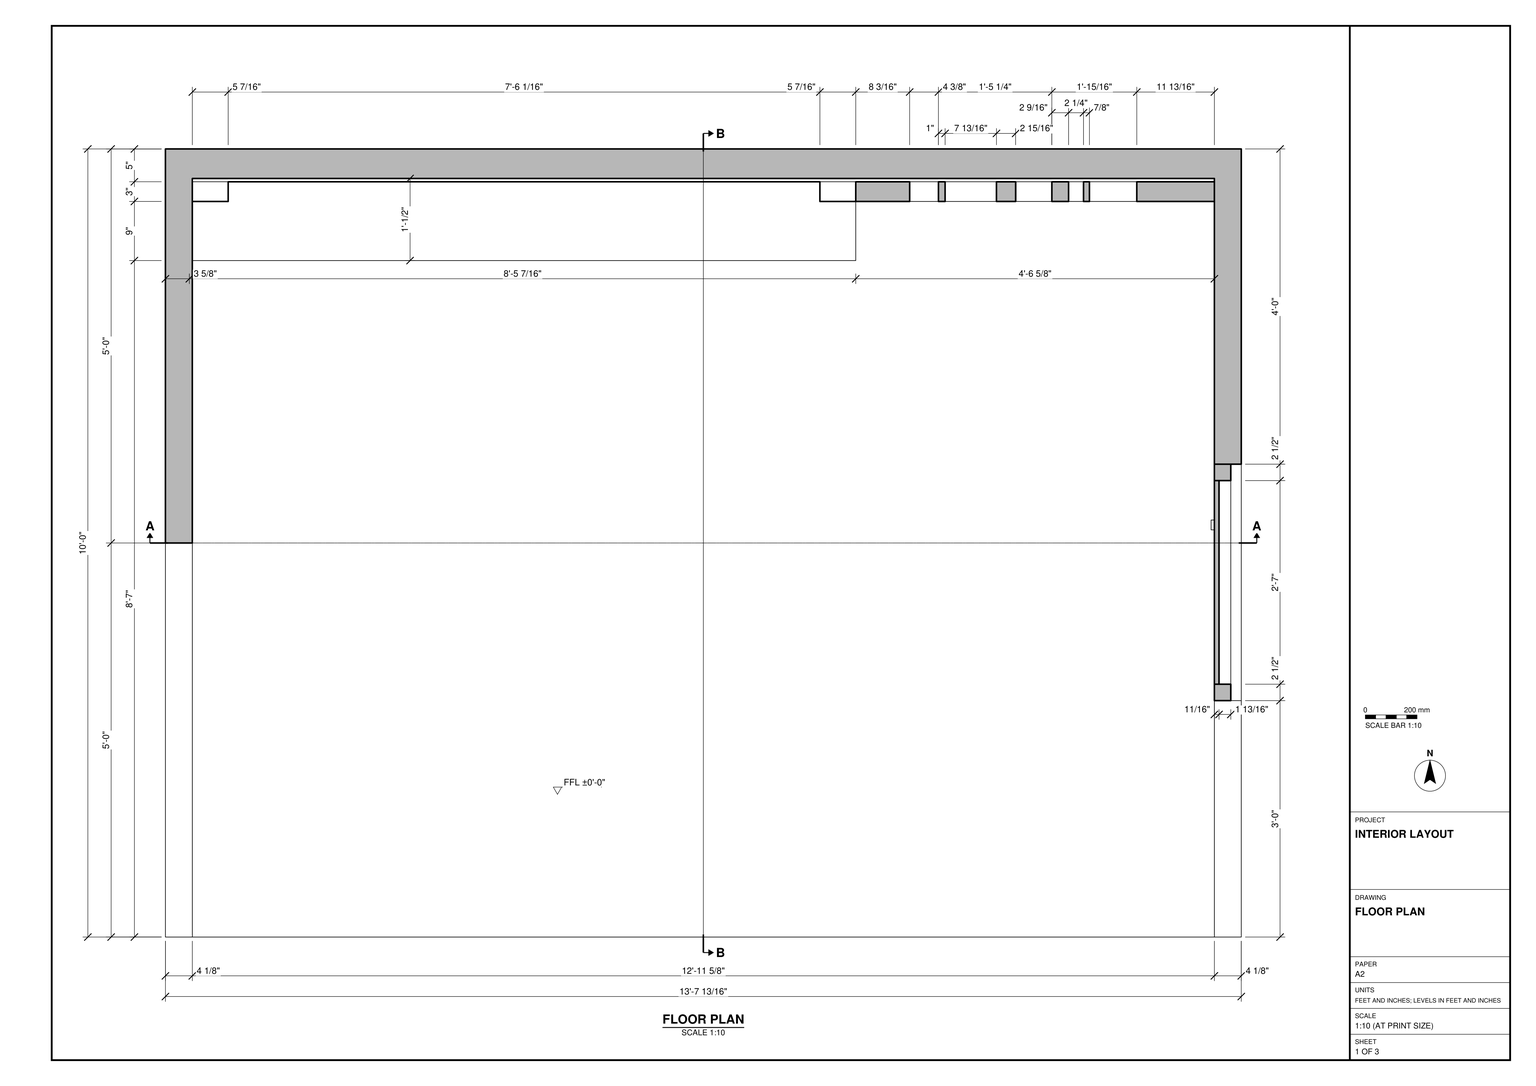
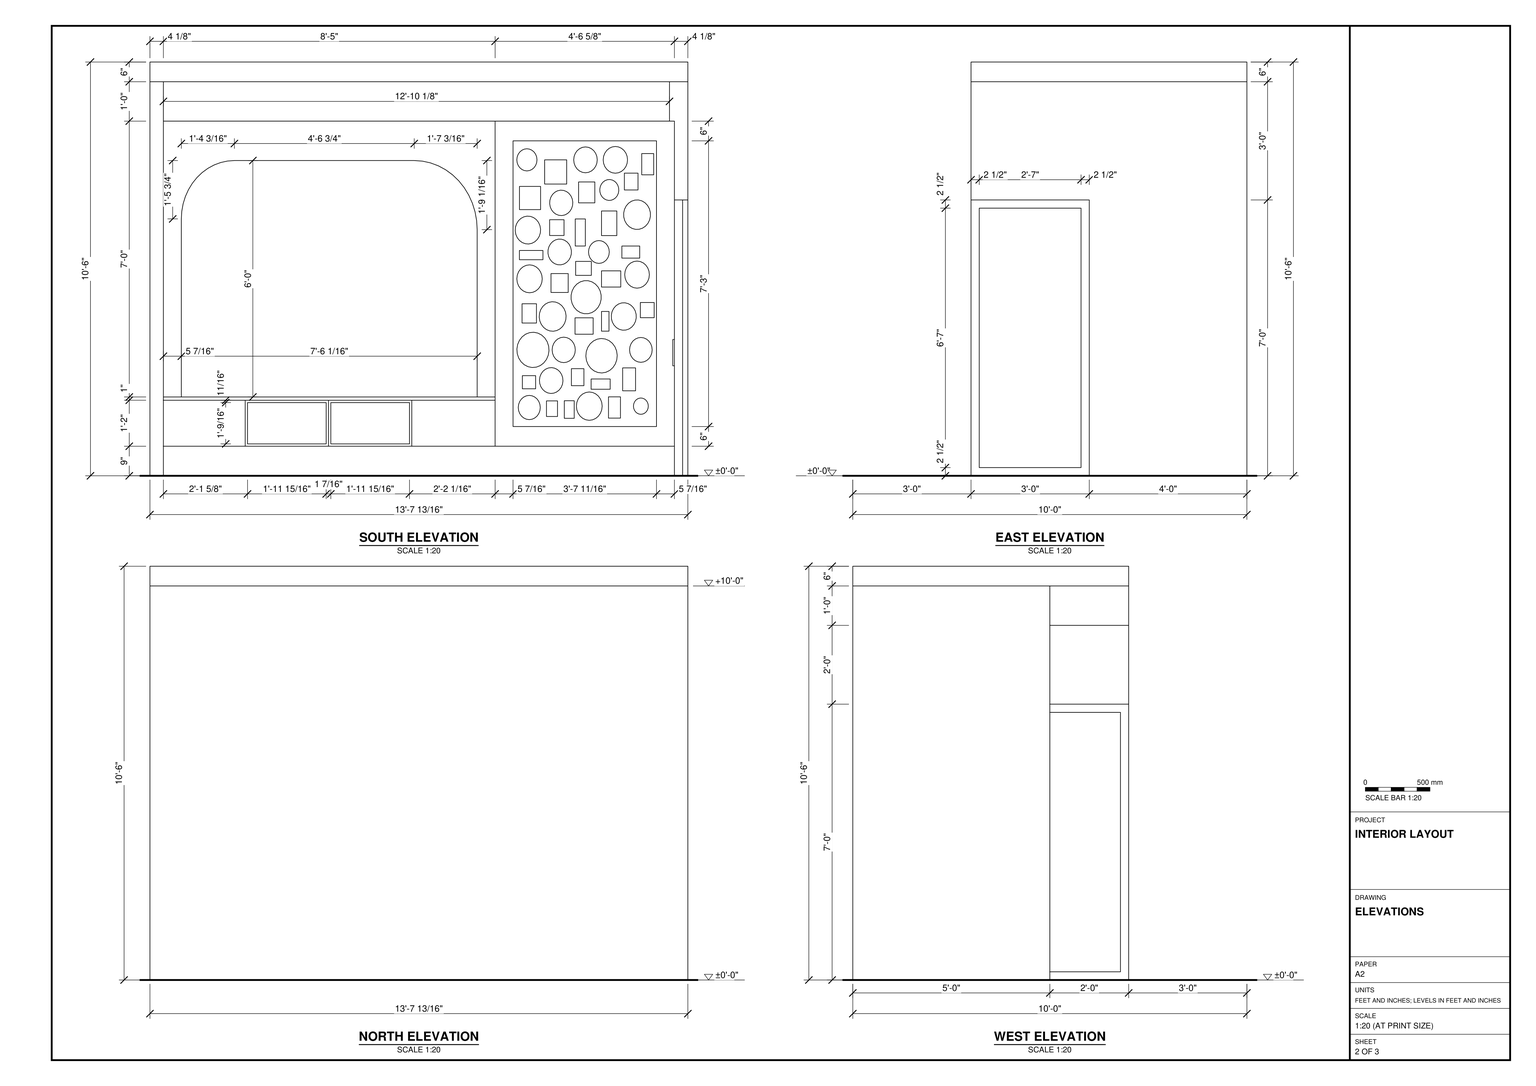
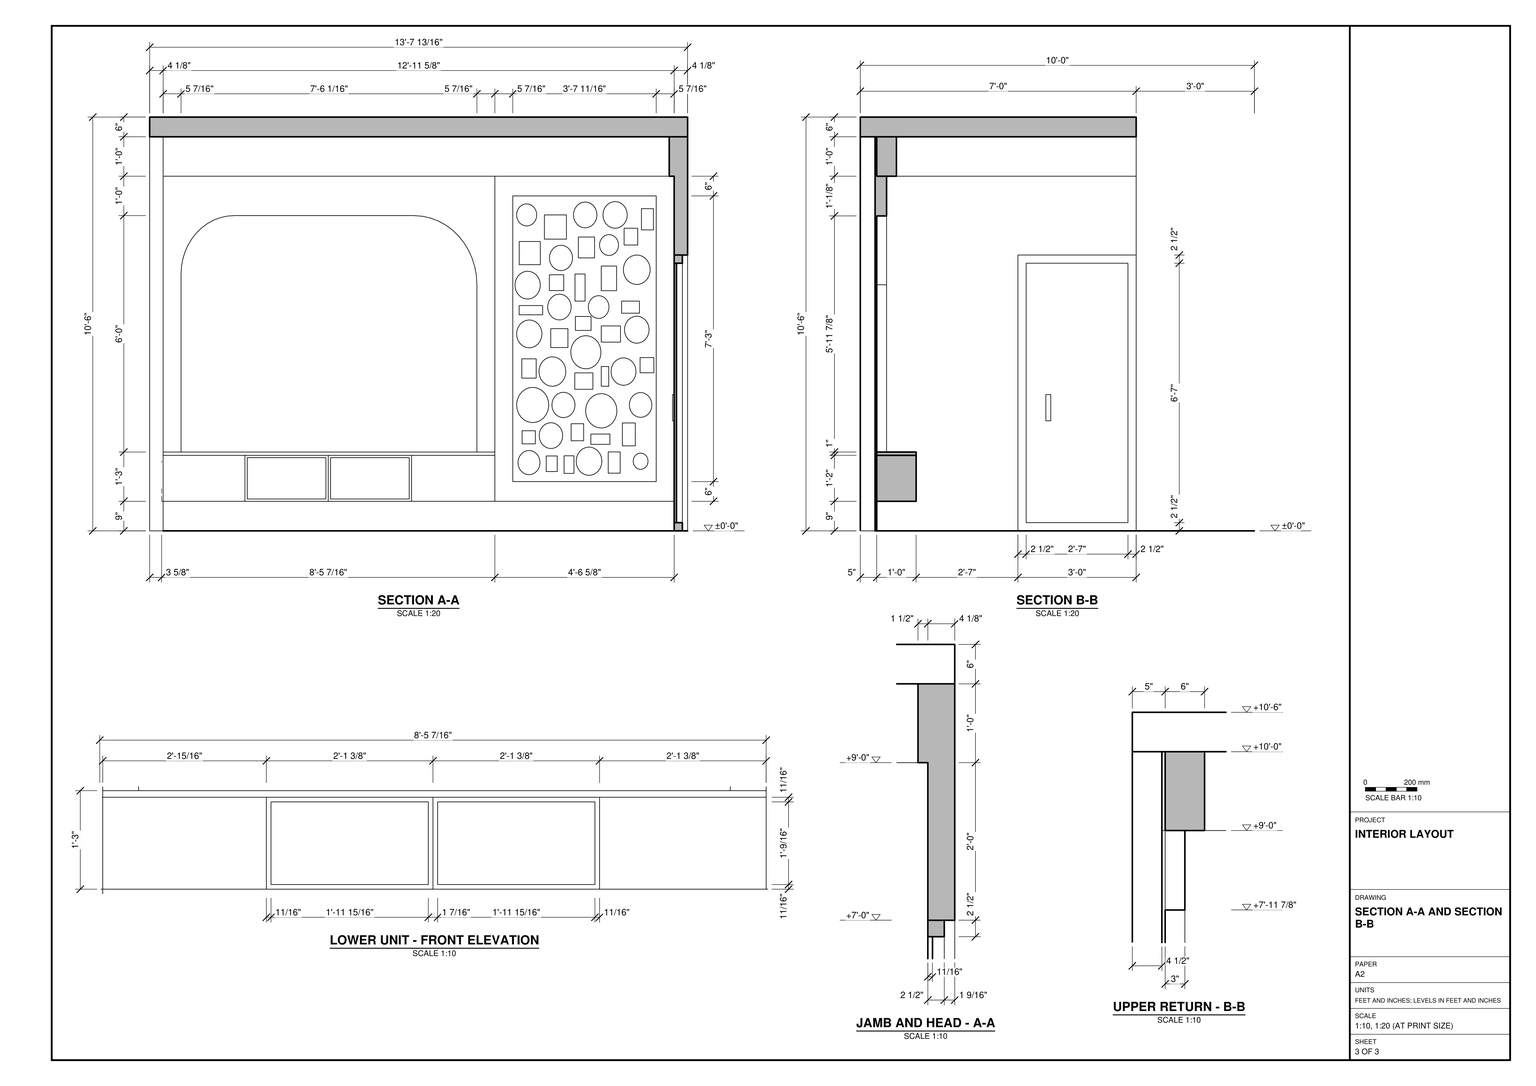
Build the interior shown in task_files/diagram_01.pdf in SketchUp. Work in feet and inches. The overall width is 13'-7 13/16", the depth is 10'-0", and the height is 10'-6". Set the finished floor at ±0'-0". Use the floor plan to lay out the back wall and its unequal side returns. Follow the wall thicknesses as drawn, leave the front open, and stop the overhead slab short of the front edge as shown in section B-B.

Use the south elevation to lay out the fitted wall. In the wider left bay, form the panel with straight sides, rounded upper corners and a horizontal head. Fit the suspended lower unit beneath it, with a continuous top, two inset rectangular fronts in the middle and plain end sections. In the narrower right bay, model the tall framed panel with the arrangement of circles and rectangles shown. Follow the sections for the depth of the joinery, the upper return and the head and jamb of the framed window in the right side wall.

Keep shell elements such as walls and slabs and each furniture or joinery piece in separate groups or components, and use components for repeated parts. Any decor or loose items may be suitable library components. Save one SketchUp model as output_files/fitted_feature_wall_with_suspended_cabinet.skp.

# SketchUp Ruby script. Lengths in inches.
U = 1.inch
M = Sketchup.active_model
def pt(a) = Geom::Point3d.new(a.map { |v| v * U })
def face(e, loops, mat)
  f = e.add_face(loops[0].map { |a| pt(a) })
  loops[1..].each { |l| e.add_face(l.map { |a| pt(a) }).erase! }
  f.material = f.back_material = mat if mat
  f
end
# faces: each face lists its corners as indices into pts; further lists are holes
def faces(e, pts, list, mat = nil) = list.each { |f| face(e, (f[0].is_a?(Array) ? f : [f]).map { |l| l.map { |i| pts[i] } }, mat) }
# xy, xz, yz: faces in a plane at the given z, y or x. An outline is a flat list of corners, or four numbers for a rectangle; further outlines are holes
def ring(l) = l.size == 4 ? [[l[0], l[1]], [l[2], l[1]], [l[2], l[3]], [l[0], l[3]]] : l.each_slice(2).to_a
def flat(e, list, mat, &to3) = list.each { |f| face(e, (f[0].is_a?(Array) ? f : [f]).map { |l| ring(l).map { |u, v| to3.(u, v) } }, mat) }
def xy(e, z, list, mat = nil) = flat(e, list, mat) { |x, y| [x, y, z] }
def xz(e, y, list, mat = nil) = flat(e, list, mat) { |x, z| [x, y, z] }
def yz(e, x, list, mat = nil) = flat(e, list, mat) { |y, z| [x, y, z] }
def lines(e, pts, list) = list.each { |a, b| e.add_line(pt(pts[a]), pt(pts[b])) }
# prism: a flat outline (further loops are holes) pulled along v
def prism(e, loops, v, mat = nil)
  f = face(e, loops, mat); d = Geom::Vector3d.new(v.map { |x| x * U })
  f.pushpull(f.normal.samedirection?(d) ? d.length : -d.length)
end
def box(e, o, s, mat = nil) = prism(e, [[o, [o[0] + s[0], o[1], o[2]], [o[0] + s[0], o[1] + s[1], o[2]], [o[0], o[1] + s[1], o[2]]]], [0, 0, s[2]], mat)
def at(x, y, z, deg = 0) = Geom::Transformation.translation(pt([x, y, z])) * Geom::Transformation.rotation(ORIGIN, Z_AXIS, deg.degrees)
def axes(o, x, y, z) = Geom::Transformation.new([*x, 0, *y, 0, *z, 0, *pt(o).to_a, 1])
def part(name) = M.definitions.add(name)
# library, detail: a bought-in or finely detailed component or shape, given as its bounding box
def library(name, o, s) = part(name).tap { |d| box(d.entities, o, s) }
def detail(e, o, s) = box(e.add_group.entities, o, s)
def put(e, d, t, mat = nil) = e.add_instance(d, t).tap { |i| i.material = mat if mat }
def group(e, t, mat = nil) = e.add_group.tap { |g| g.transformation = t; g.material = mat if mat }.entities
root = M.entities
M.materials.add("Glass Smoked 001").color = [0, 0, 0]
M.materials["Glass Smoked 001"].alpha = 0.1
M.materials.add("Marble Black 100cm").color = [32, 32, 32]
M.materials.add("Marble White 100cm").color = [222, 222, 222]
M.materials.add("Metal Sandblasted Black 200cm").color = [86, 90, 95]
M.materials.add("PVC Poised Taupe Matte Rough 001").color = [140, 135, 132]
M.materials.add("Wall Paint Fine Grain 01 Yellow 100cm").color = [207, 190, 139]
M.materials.add("Wood 13-07 100cm").color = [172, 111, 59]
M.materials.add("Wood Light 08 200cm").color = [239, 225, 202]
c1 = library("Group\#5",[0,-3,0],[60,3,99])
g1 = group(root,at(0,0,0))
xy(g1,0,[[4.1,0,159.7,0,159.7,115.5,4.09,115.5,4.1,60]],"Marble White 100cm")
xy(g1,0,[[0,0,4.1,60],[159.7,0,163.8,36],[159.7,36,163.8,72]],"Wall Paint Fine Grain 01 Yellow 100cm")
xy(g1,84,[[159.7,36,163.8,72]],"Wall Paint Fine Grain 01 Yellow 100cm")
xy(g1,108,[[158.2,36,159.7,115.5]],"Wall Paint Fine Grain 01 Yellow 100cm")
xy(g1,120,[[158.2,36,163.8,36,163.8,120,0,120,0,60,4.1,60,4.09,115.5,158.2,115.5]],"Wall Paint Fine Grain 01 Yellow 100cm")
xz(g1,36,[[159.7,84,163.8,84,163.8,120,158.2,120,158.2,108,159.7,108]],"Wall Paint Fine Grain 01 Yellow 100cm")
xz(g1,60,[[0,0,4.1,120]],"Wall Paint Fine Grain 01 Yellow 100cm")
xz(g1,72,[[159.7,0,163.8,84]],"Wall Paint Fine Grain 01 Yellow 100cm")
xz(g1,115.5,[[4.09,0,159.7,0,159.7,108,158.2,108,158.2,120,4.09,120]],"Wall Paint Fine Grain 01 Yellow 100cm")
xz(g1,120,[[0,0,163.8,120]],"Wall Paint Fine Grain 01 Yellow 100cm")
yz(g1,0,[[60,0,120,120]],"Wall Paint Fine Grain 01 Yellow 100cm")
yz(g1,158.2,[[36,108,115.5,120]],"Wall Paint Fine Grain 01 Yellow 100cm")
yz(g1,159.7,[[72,0,72,84,36,84,36,108,115.5,108,115.5,0]],"Wall Paint Fine Grain 01 Yellow 100cm")
yz(g1,163.8,[[72,0,120,0,120,120,36,120,36,84,72,84]],"Wall Paint Fine Grain 01 Yellow 100cm")
p = [[4.1,60,0],[4.09,115.5,0],[4.09,115.5,120],[4.1,60,120]]
faces(g1,p,[[0,1,2,3]],"Wall Paint Fine Grain 01 Yellow 100cm")
g2 = group(g1,at(159.7,36,0))
prism(g2,[[[0,36,84],[0,36,0],[0,0,0],[0,0,84]],[[0,2.5,2.5],[0,33.5,2.5],[0,33.5,81.5],[0,2.5,81.5]]],[2.5,0,0],"Metal Sandblasted Black 200cm")
g3 = group(g2,at(0,2.5,2.5))
box(g3,[0,0,0],[0.71,31,79],"Wood 13-07 100cm")
g4 = group(g1,at(159.7,62,33.5))
box(g4,[-0.5,0,0],[0.5,1.5,8],"Metal Sandblasted Black 200cm")
g5 = group(root,at(4.09,115.5,0))
xy(g5,0,[[0,-0.5,155.61,0]],"Wall Paint Fine Grain 01 Yellow 100cm")
xy(g5,24,[[0,-3.5,5.46,-0.5],[95.55,-3.5,101.01,-0.5]],"Wall Paint Fine Grain 01 Yellow 100cm")
xy(g5,96,[[21.625,-3.5,76.38,-0.5]],"Wall Paint Fine Grain 01 Yellow 100cm")
xy(g5,108,[[0,-3.5,101.01,-0.5]],"Wall Paint Fine Grain 01 Yellow 100cm")
xy(g5,120,[[0,-0.5,155.61,0]],"Wall Paint Fine Grain 01 Yellow 100cm")
xz(g5,-3.5,[[0,24,5.46,24,5.46,78.24,5.6,80.55,6.01,82.83,6.69,85.03,7.625,87.12,8.8,89.05,10.19,90.8,11.78,92.33,13.54,93.62,15.4375,94.65,17.44,95.39,19.52,95.85,21.625,96,76.38,96,78.89,95.82,81.35,95.28,83.72,94.4,85.97,93.18,88.05,91.65,89.9375,89.83,91.59,87.76,92.98,85.47,94.09,83,94.9,80.39,95.39,77.6875,95.55,74.9375,95.55,24,101.01,24,101.01,108,0,108]],"Wall Paint Fine Grain 01 Yellow 100cm")
xz(g5,-0.5,[[5.46,24,95.55,24,95.55,74.9375,95.39,77.6875,94.9,80.39,94.09,83,92.98,85.47,91.59,87.76,89.9375,89.83,88.05,91.65,85.97,93.18,83.72,94.4,81.35,95.28,78.89,95.82,76.38,96,21.625,96,19.52,95.85,17.44,95.39,15.4375,94.65,13.54,93.62,11.78,92.33,10.19,90.8,8.8,89.05,7.625,87.12,6.69,85.03,6.01,82.83,5.6,80.55,5.46,78.24]],"Marble Black 100cm")
xz(g5,-0.5,[[0,0,155.61,0,155.61,9,101.01,9,101.01,24,95.55,24,95.55,23,5.46,23,5.46,24,0,24],[0,108,155.61,120]],"Wall Paint Fine Grain 01 Yellow 100cm")
xz(g5,0,[[0,0,155.61,120]],"Wall Paint Fine Grain 01 Yellow 100cm")
yz(g5,0,[[-0.5,0,-0.5,24,-3.5,24,-3.5,108,-0.5,108,-0.5,120,0,120,0,0]],"Wall Paint Fine Grain 01 Yellow 100cm")
yz(g5,5.46,[[-3.5,24,-0.5,78.24]],"Wall Paint Fine Grain 01 Yellow 100cm")
yz(g5,95.55,[[-3.5,24,-0.5,74.9375]],"Wall Paint Fine Grain 01 Yellow 100cm")
yz(g5,101.01,[[-3.5,24,-0.5,108]],"Wall Paint Fine Grain 01 Yellow 100cm")
yz(g5,155.61,[[-0.5,0,0,120]],"Wall Paint Fine Grain 01 Yellow 100cm")
p = [[95.39,-0.5,77.6875],[95.55,-0.5,74.9375],[95.55,-3.5,74.9375],[95.39,-3.5,77.6875],[94.9,-0.5,80.39],[94.9,-3.5,80.39],
  [5.46,-0.5,78.24],[5.6,-0.5,80.55],[5.6,-3.5,80.55],[5.46,-3.5,78.24],[94.09,-0.5,83],[94.09,-3.5,83],
  [6.01,-0.5,82.83],[6.01,-3.5,82.83],[6.69,-0.5,85.03],[6.69,-3.5,85.03],[92.98,-0.5,85.47],[92.98,-3.5,85.47],
  [7.625,-0.5,87.12],[7.625,-3.5,87.12],[91.59,-0.5,87.76],[91.59,-3.5,87.76],[8.8,-0.5,89.05],[8.8,-3.5,89.05],
  [89.9375,-0.5,89.83],[89.9375,-3.5,89.83],[10.19,-0.5,90.8],[10.19,-3.5,90.8],[88.05,-0.5,91.65],[88.05,-3.5,91.65],
  [11.78,-0.5,92.33],[11.78,-3.5,92.33],[85.97,-0.5,93.18],[85.97,-3.5,93.18],[13.54,-0.5,93.62],[13.54,-3.5,93.62],
  [83.72,-0.5,94.4],[83.72,-3.5,94.4],[15.4375,-0.5,94.65],[15.4375,-3.5,94.65],[81.35,-0.5,95.28],[81.35,-3.5,95.28],
  [17.44,-0.5,95.39],[17.44,-3.5,95.39],[78.89,-0.5,95.82],[78.89,-3.5,95.82],[19.52,-0.5,95.85],[19.52,-3.5,95.85],
  [21.625,-0.5,96],[21.625,-3.5,96],[76.38,-0.5,96],[76.38,-3.5,96]]
faces(g5,p,[[0,1,2,3],[4,0,3,5],[6,7,8,9],[10,4,5,11],[7,12,13,8],[12,14,15,13],[16,10,11,17],[14,18,19,15],
  [20,16,17,21],[18,22,23,19],[24,20,21,25],[22,26,27,23],[28,24,25,29],[26,30,31,27],[32,28,29,33],[30,34,35,31],
  [36,32,33,37],[34,38,39,35],[40,36,37,41],[38,42,43,39],[44,40,41,45],[42,46,47,43],[46,48,49,47],[50,44,45,51]],"Wall Paint Fine Grain 01 Yellow 100cm")
g6 = group(g5,at(5.46,-0.5,9))
xy(g6,0,[[-5.92,-12,95.55,0]])
xy(g6,0.71,[[20.16,-12,44.11,-1],[45.53,-12,69.48,-1.0625]],"PVC Poised Taupe Matte Rough 001")
xy(g6,13.29,[[20.16,-12,44.11,-1],[45.53,-12,69.48,-1.0625]],"PVC Poised Taupe Matte Rough 001")
xy(g6,14,[[-5.92,-12,95.55,0]])
xz(g6,-12,[[[19.45,0,44.82,14],[20.16,0.71,44.11,13.29]],[[44.82,0,70.18,14],[45.53,0.71,69.48,13.29]]],"Metal Sandblasted Black 200cm")
xz(g6,-12,[[-5.92,0,19.45,14],[70.18,0,95.55,14]],"Wood Light 08 200cm")
xz(g6,-1.0625,[[45.53,0.71,69.48,13.29]],"PVC Poised Taupe Matte Rough 001")
xz(g6,-1,[[20.16,0.71,44.11,13.29]],"PVC Poised Taupe Matte Rough 001")
xz(g6,0,[[-5.92,0,95.55,14]])
yz(g6,-5.92,[[-12,0,0,14]])
yz(g6,20.16,[[-12,0.71,-1,13.29]],"PVC Poised Taupe Matte Rough 001")
yz(g6,44.11,[[-12,0.71,-1,13.29]],"PVC Poised Taupe Matte Rough 001")
yz(g6,45.53,[[-12,0.71,-1.0625,13.29]],"PVC Poised Taupe Matte Rough 001")
yz(g6,69.48,[[-12,0.71,-1.0625,13.29]],"PVC Poised Taupe Matte Rough 001")
yz(g6,95.55,[[-12,0,0,14]],"Wood Light 08 200cm")
g7 = group(g5,at(5.46,-0.5,23),"Wood 13-07 100cm")
box(g7,[-5.46,-12,0],[101.01,12,1],"Wood 13-07 100cm")
put(g5,c1,axes([101.01,-0.5,9],[0.91,0,0],[0,1,0],[0,0,1]),"Wood 13-07 100cm")
g8 = group(g5,at(25.62,-12.5,9.71),"Glass Smoked 001")
box(g8,[0,0,0],[23.95,0.31,12.58])
g9 = group(g5,at(50.99,-12.5,9.71),"Glass Smoked 001")
box(g9,[0,0,0],[23.95,0.31,12.58])
g10 = group(root,at(4.09,115,108),"Wall Paint Fine Grain 01 Yellow 100cm")
box(g10,[0,-6,0],[155.61,6,12],"Wall Paint Fine Grain 01 Yellow 100cm")
g11 = group(root,at(0,36,120))
box(g11,[0,0,0],[163.8,84,6])
